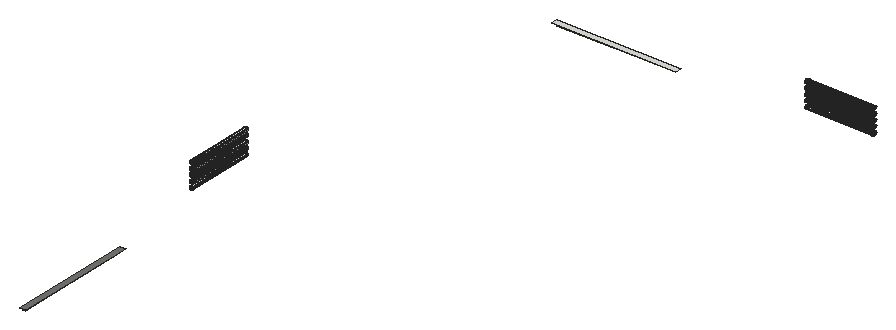
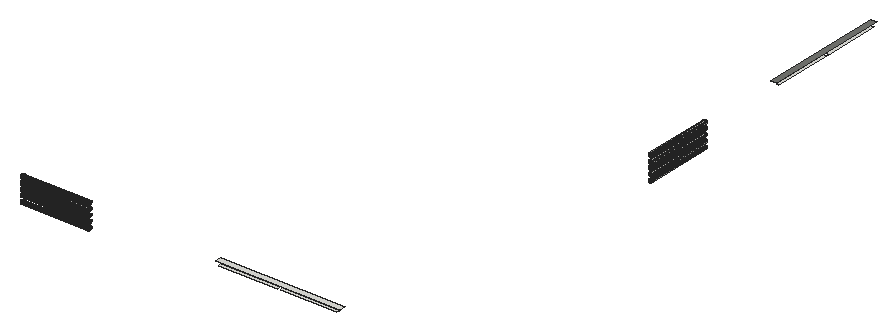
# SketchUp Ruby script. Lengths in inches.
U = 1.inch
M = Sketchup.active_model
def pt(a) = Geom::Point3d.new(a.map { |v| v * U })
def face(e, loops, mat)
  f = e.add_face(loops[0].map { |a| pt(a) })
  loops[1..].each { |l| e.add_face(l.map { |a| pt(a) }).erase! }
  f.material = f.back_material = mat if mat
  f
end
# faces: each face lists its corners as indices into pts; further lists are holes
def faces(e, pts, list, mat = nil) = list.each { |f| face(e, (f[0].is_a?(Array) ? f : [f]).map { |l| l.map { |i| pts[i] } }, mat) }
# xy, xz, yz: faces in a plane at the given z, y or x. An outline is a flat list of corners, or four numbers for a rectangle; further outlines are holes
def ring(l) = l.size == 4 ? [[l[0], l[1]], [l[2], l[1]], [l[2], l[3]], [l[0], l[3]]] : l.each_slice(2).to_a
def flat(e, list, mat, &to3) = list.each { |f| face(e, (f[0].is_a?(Array) ? f : [f]).map { |l| ring(l).map { |u, v| to3.(u, v) } }, mat) }
def xy(e, z, list, mat = nil) = flat(e, list, mat) { |x, y| [x, y, z] }
def xz(e, y, list, mat = nil) = flat(e, list, mat) { |x, z| [x, y, z] }
def yz(e, x, list, mat = nil) = flat(e, list, mat) { |y, z| [x, y, z] }
def lines(e, pts, list) = list.each { |a, b| e.add_line(pt(pts[a]), pt(pts[b])) }
# prism: a flat outline (further loops are holes) pulled along v
def prism(e, loops, v, mat = nil)
  f = face(e, loops, mat); d = Geom::Vector3d.new(v.map { |x| x * U })
  f.pushpull(f.normal.samedirection?(d) ? d.length : -d.length)
end
def box(e, o, s, mat = nil) = prism(e, [[o, [o[0] + s[0], o[1], o[2]], [o[0] + s[0], o[1] + s[1], o[2]], [o[0], o[1] + s[1], o[2]]]], [0, 0, s[2]], mat)
def at(x, y, z, deg = 0) = Geom::Transformation.translation(pt([x, y, z])) * Geom::Transformation.rotation(ORIGIN, Z_AXIS, deg.degrees)
def axes(o, x, y, z) = Geom::Transformation.new([*x, 0, *y, 0, *z, 0, *pt(o).to_a, 1])
def part(name) = M.definitions.add(name)
# library, detail: a bought-in or finely detailed component or shape, given as its bounding box
def library(name, o, s) = part(name).tap { |d| box(d.entities, o, s) }
def detail(e, o, s) = box(e.add_group.entities, o, s)
def put(e, d, t, mat = nil) = e.add_instance(d, t).tap { |i| i.material = mat if mat }
def group(e, t, mat = nil) = e.add_group.tap { |g| g.transformation = t; g.material = mat if mat }.entities
root = M.entities
M.materials.add("[Metal Seamed]").color = [118, 119, 115]
xy(root,1727.61,[[120,175.92,126,293.77],[120,299.77,126,423.61],[211.11,1458.8125,328.96,1464.8125],[334.96,1458.8125,458.8,1464.8125]])
xy(root,1733.61,[[205.11,1452.8125,464.8,1464.8125]])
xy(root,1733.61,[[120,169.92,132,429.61]],"[Metal Seamed]")
p = [[83.53,662.8,1725.02],[82.57,662.8,1725.14],[82.57,806.17,1725.14],[83.53,806.17,1725.02],[84.48,662.8,1725.14],[84.48,806.17,1725.14],
  [697.99,1500.33,1725.14],[697.99,1501.28,1725.02],[841.36,1501.28,1725.02],[841.36,1500.33,1725.14],[697.99,1502.24,1725.14],[841.36,1502.24,1725.14],
  [81.68,662.8,1725.51],[81.68,806.17,1725.51],[85.37,662.8,1725.51],[85.37,806.17,1725.51],[697.99,1499.44,1725.51],[841.36,1499.44,1725.51],
  [697.99,1503.13,1725.51],[841.36,1503.13,1725.51],[80.92,662.8,1726.1],[80.92,806.17,1726.1],[86.13,662.8,1726.1],[86.13,806.17,1726.1],
  [697.99,1498.68,1726.1],[841.36,1498.68,1726.1],[697.99,1503.89,1726.1],[841.36,1503.89,1726.1],[80.33,662.8,1726.86],[80.33,806.17,1726.86],
  [86.72,662.8,1726.86],[86.72,806.17,1726.86],[697.99,1498.09,1726.86],[841.36,1498.09,1726.86],[697.99,1504.48,1726.86],[841.36,1504.48,1726.86],
  [79.97,662.8,1727.75],[79.97,806.17,1727.75],[87.09,662.8,1727.75],[87.09,806.17,1727.75],[697.99,1497.72,1727.75],[841.36,1497.72,1727.75],
  [697.99,1504.85,1727.75],[841.36,1504.85,1727.75],[79.84,662.8,1728.7],[79.84,806.17,1728.7],[87.21,662.8,1728.7],[87.21,806.17,1728.7],
  [697.99,1497.6,1728.7],[841.36,1497.6,1728.7],[697.99,1504.97,1728.7],[841.36,1504.97,1728.7],[79.97,662.8,1729.66],[79.97,806.17,1729.66],
  [87.09,662.8,1729.66],[87.09,806.17,1729.66],[697.99,1497.72,1729.66],[841.36,1497.72,1729.66],[697.99,1504.85,1729.66],[841.36,1504.85,1729.66],
  [80.33,662.8,1730.55],[80.33,806.17,1730.55],[86.72,662.8,1730.55],[86.72,806.17,1730.55],[697.99,1498.09,1730.55],[841.36,1498.09,1730.55],
  [697.99,1504.48,1730.55],[841.36,1504.48,1730.55],[80.92,662.8,1731.3125],[80.92,806.17,1731.3125],[86.13,662.8,1731.3125],[86.13,806.17,1731.3125],
  [697.99,1498.68,1731.3125],[841.36,1498.68,1731.3125],[697.99,1503.89,1731.3125],[841.36,1503.89,1731.3125],[81.68,662.8,1731.9],[81.68,806.17,1731.9],
  [85.37,662.8,1731.9],[85.37,806.17,1731.9],[697.99,1499.44,1731.9],[841.36,1499.44,1731.9],[697.99,1503.13,1731.9],[841.36,1503.13,1731.9],
  [82.57,662.8,1732.27],[82.57,806.17,1732.27],[84.48,662.8,1732.27],[84.48,806.17,1732.27],[697.99,1500.33,1732.27],[841.36,1500.33,1732.27],
  [697.99,1502.24,1732.27],[841.36,1502.24,1732.27],[83.53,662.8,1732.39],[83.53,806.17,1732.39],[697.99,1501.28,1732.39],[841.36,1501.28,1732.39],
  [83.53,662.8,1737.02],[82.57,662.8,1737.14],[82.57,806.17,1737.14],[83.53,806.17,1737.02],[84.48,662.8,1737.14],[84.48,806.17,1737.14],
  [697.99,1500.33,1737.14],[697.99,1501.28,1737.02],[841.36,1501.28,1737.02],[841.36,1500.33,1737.14],[697.99,1502.24,1737.14],[841.36,1502.24,1737.14],
  [81.68,662.8,1737.51],[81.68,806.17,1737.51],[85.37,662.8,1737.51],[85.37,806.17,1737.51],[697.99,1499.44,1737.51],[841.36,1499.44,1737.51],
  [697.99,1503.13,1737.51],[841.36,1503.13,1737.51],[80.92,662.8,1738.1],[80.92,806.17,1738.1],[86.13,662.8,1738.1],[86.13,806.17,1738.1],
  [697.99,1498.68,1738.1],[841.36,1498.68,1738.1],[697.99,1503.89,1738.1],[841.36,1503.89,1738.1],[80.33,662.8,1738.86],[80.33,806.17,1738.86],
  [86.72,662.8,1738.86],[86.72,806.17,1738.86],[697.99,1498.09,1738.86],[841.36,1498.09,1738.86],[697.99,1504.48,1738.86],[841.36,1504.48,1738.86],
  [79.97,662.8,1739.75],[79.97,806.17,1739.75],[87.09,662.8,1739.75],[87.09,806.17,1739.75],[697.99,1497.72,1739.75],[841.36,1497.72,1739.75],
  [697.99,1504.85,1739.75],[841.36,1504.85,1739.75],[79.84,662.8,1740.7],[79.84,806.17,1740.7],[87.21,662.8,1740.7],[87.21,806.17,1740.7],
  [697.99,1497.6,1740.7],[841.36,1497.6,1740.7],[697.99,1504.97,1740.7],[841.36,1504.97,1740.7],[79.97,662.8,1741.66],[79.97,806.17,1741.66],
  [87.09,662.8,1741.66],[87.09,806.17,1741.66],[697.99,1497.72,1741.66],[841.36,1497.72,1741.66],[697.99,1504.85,1741.66],[841.36,1504.85,1741.66],
  [80.33,662.8,1742.55],[80.33,806.17,1742.55],[86.72,662.8,1742.55],[86.72,806.17,1742.55],[697.99,1498.09,1742.55],[841.36,1498.09,1742.55],
  [697.99,1504.48,1742.55],[841.36,1504.48,1742.55],[80.92,662.8,1743.3125],[80.92,806.17,1743.3125],[86.13,662.8,1743.3125],[86.13,806.17,1743.3125],
  [697.99,1498.68,1743.3125],[841.36,1498.68,1743.3125],[697.99,1503.89,1743.3125],[841.36,1503.89,1743.3125],[81.68,662.8,1743.9],[81.68,806.17,1743.9],
  [85.37,662.8,1743.9],[85.37,806.17,1743.9],[697.99,1499.44,1743.9],[841.36,1499.44,1743.9],[697.99,1503.13,1743.9],[841.36,1503.13,1743.9],
  [82.57,662.8,1744.27],[82.57,806.17,1744.27],[84.48,662.8,1744.27],[84.48,806.17,1744.27],[697.99,1500.33,1744.27],[841.36,1500.33,1744.27],
  [697.99,1502.24,1744.27],[841.36,1502.24,1744.27],[83.53,662.8,1744.39],[83.53,806.17,1744.39],[697.99,1501.28,1744.39],[841.36,1501.28,1744.39],
  [83.53,662.8,1749.02],[82.57,662.8,1749.14],[82.57,806.17,1749.14],[83.53,806.17,1749.02],[84.48,662.8,1749.14],[84.48,806.17,1749.14],
  [697.99,1500.33,1749.14],[697.99,1501.28,1749.02],[841.36,1501.28,1749.02],[841.36,1500.33,1749.14],[697.99,1502.24,1749.14],[841.36,1502.24,1749.14],
  [81.68,662.8,1749.51],[81.68,806.17,1749.51],[85.37,662.8,1749.51],[85.37,806.17,1749.51],[697.99,1499.44,1749.51],[841.36,1499.44,1749.51],
  [697.99,1503.13,1749.51],[841.36,1503.13,1749.51],[80.92,662.8,1750.1],[80.92,806.17,1750.1],[86.13,662.8,1750.1],[86.13,806.17,1750.1],
  [697.99,1498.68,1750.1],[841.36,1498.68,1750.1],[697.99,1503.89,1750.1],[841.36,1503.89,1750.1],[80.33,662.8,1750.86],[80.33,806.17,1750.86],
  [86.72,662.8,1750.86],[86.72,806.17,1750.86],[697.99,1498.09,1750.86],[841.36,1498.09,1750.86],[697.99,1504.48,1750.86],[841.36,1504.48,1750.86],
  [79.97,662.8,1751.75],[79.97,806.17,1751.75],[87.09,662.8,1751.75],[87.09,806.17,1751.75],[697.99,1497.72,1751.75],[841.36,1497.72,1751.75],
  [697.99,1504.85,1751.75],[841.36,1504.85,1751.75],[79.84,662.8,1752.7],[79.84,806.17,1752.7],[87.21,662.8,1752.7],[87.21,806.17,1752.7],
  [697.99,1497.6,1752.7],[841.36,1497.6,1752.7],[697.99,1504.97,1752.7],[841.36,1504.97,1752.7],[79.97,662.8,1753.66],[79.97,806.17,1753.66],
  [87.09,662.8,1753.66],[87.09,806.17,1753.66],[697.99,1497.72,1753.66],[841.36,1497.72,1753.66],[697.99,1504.85,1753.66],[841.36,1504.85,1753.66],
  [80.33,662.8,1754.55],[80.33,806.17,1754.55],[86.72,662.8,1754.55],[86.72,806.17,1754.55],[697.99,1498.09,1754.55],[841.36,1498.09,1754.55],
  [697.99,1504.48,1754.55],[841.36,1504.48,1754.55],[80.92,662.8,1755.3125],[80.92,806.17,1755.3125],[86.13,662.8,1755.3125],[86.13,806.17,1755.3125],
  [697.99,1498.68,1755.3125],[841.36,1498.68,1755.3125],[697.99,1503.89,1755.3125],[841.36,1503.89,1755.3125],[81.68,662.8,1755.9],[81.68,806.17,1755.9],
  [85.37,662.8,1755.9],[85.37,806.17,1755.9],[697.99,1499.44,1755.9],[841.36,1499.44,1755.9],[697.99,1503.13,1755.9],[841.36,1503.13,1755.9],
  [82.57,662.8,1756.27],[82.57,806.17,1756.27],[84.48,662.8,1756.27],[84.48,806.17,1756.27],[697.99,1500.33,1756.27],[841.36,1500.33,1756.27],
  [697.99,1502.24,1756.27],[841.36,1502.24,1756.27],[83.53,662.8,1756.39],[83.53,806.17,1756.39],[697.99,1501.28,1756.39],[841.36,1501.28,1756.39],
  [83.53,662.8,1761.02],[82.57,662.8,1761.14],[82.57,806.17,1761.14],[83.53,806.17,1761.02],[84.48,662.8,1761.14],[84.48,806.17,1761.14],
  [697.99,1500.33,1761.14],[697.99,1501.28,1761.02],[841.36,1501.28,1761.02],[841.36,1500.33,1761.14],[697.99,1502.24,1761.14],[841.36,1502.24,1761.14],
  [81.68,662.8,1761.51],[81.68,806.17,1761.51],[85.37,662.8,1761.51],[85.37,806.17,1761.51],[697.99,1499.44,1761.51],[841.36,1499.44,1761.51],
  [697.99,1503.13,1761.51],[841.36,1503.13,1761.51],[80.92,662.8,1762.1],[80.92,806.17,1762.1],[86.13,662.8,1762.1],[86.13,806.17,1762.1],
  [697.99,1498.68,1762.1],[841.36,1498.68,1762.1],[697.99,1503.89,1762.1],[841.36,1503.89,1762.1],[80.33,662.8,1762.86],[80.33,806.17,1762.86],
  [86.72,662.8,1762.86],[86.72,806.17,1762.86],[697.99,1498.09,1762.86],[841.36,1498.09,1762.86],[697.99,1504.48,1762.86],[841.36,1504.48,1762.86],
  [79.97,662.8,1763.75],[79.97,806.17,1763.75],[87.09,662.8,1763.75],[87.09,806.17,1763.75],[697.99,1497.72,1763.75],[841.36,1497.72,1763.75],
  [697.99,1504.85,1763.75],[841.36,1504.85,1763.75],[79.84,662.8,1764.7],[79.84,806.17,1764.7],[87.21,662.8,1764.7],[87.21,806.17,1764.7],
  [697.99,1497.6,1764.7],[841.36,1497.6,1764.7],[697.99,1504.97,1764.7],[841.36,1504.97,1764.7],[79.97,662.8,1765.66],[79.97,806.17,1765.66],
  [87.09,662.8,1765.66],[87.09,806.17,1765.66],[697.99,1497.72,1765.66],[841.36,1497.72,1765.66],[697.99,1504.85,1765.66],[841.36,1504.85,1765.66],
  [80.33,662.8,1766.55],[80.33,806.17,1766.55],[86.72,662.8,1766.55],[86.72,806.17,1766.55],[697.99,1498.09,1766.55],[841.36,1498.09,1766.55],
  [697.99,1504.48,1766.55],[841.36,1504.48,1766.55],[80.92,662.8,1767.3125],[80.92,806.17,1767.3125],[86.13,662.8,1767.3125],[86.13,806.17,1767.3125],
  [697.99,1498.68,1767.3125],[841.36,1498.68,1767.3125],[697.99,1503.89,1767.3125],[841.36,1503.89,1767.3125],[81.68,662.8,1767.9],[81.68,806.17,1767.9],
  [85.37,662.8,1767.9],[85.37,806.17,1767.9],[697.99,1499.44,1767.9],[841.36,1499.44,1767.9],[697.99,1503.13,1767.9],[841.36,1503.13,1767.9],
  [82.57,662.8,1768.27],[82.57,806.17,1768.27],[84.48,662.8,1768.27],[84.48,806.17,1768.27],[697.99,1500.33,1768.27],[841.36,1500.33,1768.27],
  [697.99,1502.24,1768.27],[841.36,1502.24,1768.27],[83.53,662.8,1768.39],[83.53,806.17,1768.39],[697.99,1501.28,1768.39],[841.36,1501.28,1768.39],
  [83.53,662.8,1773.02],[82.57,662.8,1773.14],[82.57,806.17,1773.14],[83.53,806.17,1773.02],[84.48,662.8,1773.14],[84.48,806.17,1773.14],
  [697.99,1500.33,1773.14],[697.99,1501.28,1773.02],[841.36,1501.28,1773.02],[841.36,1500.33,1773.14],[697.99,1502.24,1773.14],[841.36,1502.24,1773.14],
  [81.68,662.8,1773.51],[81.68,806.17,1773.51],[85.37,662.8,1773.51],[85.37,806.17,1773.51],[697.99,1499.44,1773.51],[841.36,1499.44,1773.51],
  [697.99,1503.13,1773.51],[841.36,1503.13,1773.51],[80.92,662.8,1774.1],[80.92,806.17,1774.1],[86.13,662.8,1774.1],[86.13,806.17,1774.1],
  [697.99,1498.68,1774.1],[841.36,1498.68,1774.1],[697.99,1503.89,1774.1],[841.36,1503.89,1774.1],[80.33,662.8,1774.86],[80.33,806.17,1774.86],
  [86.72,662.8,1774.86],[86.72,806.17,1774.86],[697.99,1498.09,1774.86],[841.36,1498.09,1774.86],[697.99,1504.48,1774.86],[841.36,1504.48,1774.86],
  [79.97,662.8,1775.75],[79.97,806.17,1775.75],[87.09,662.8,1775.75],[87.09,806.17,1775.75],[697.99,1497.72,1775.75],[841.36,1497.72,1775.75],
  [697.99,1504.85,1775.75],[841.36,1504.85,1775.75],[79.84,662.8,1776.7],[79.84,806.17,1776.7],[87.21,662.8,1776.7],[87.21,806.17,1776.7],
  [697.99,1497.6,1776.7],[841.36,1497.6,1776.7],[697.99,1504.97,1776.7],[841.36,1504.97,1776.7],[79.97,662.8,1777.66],[79.97,806.17,1777.66],
  [87.09,662.8,1777.66],[87.09,806.17,1777.66],[697.99,1497.72,1777.66],[841.36,1497.72,1777.66],[697.99,1504.85,1777.66],[841.36,1504.85,1777.66],
  [80.33,662.8,1778.55],[80.33,806.17,1778.55],[86.72,662.8,1778.55],[86.72,806.17,1778.55],[697.99,1498.09,1778.55],[841.36,1498.09,1778.55],
  [697.99,1504.48,1778.55],[841.36,1504.48,1778.55],[80.92,662.8,1779.3125],[80.92,806.17,1779.3125],[86.13,662.8,1779.3125],[86.13,806.17,1779.3125],
  [697.99,1498.68,1779.3125],[841.36,1498.68,1779.3125],[697.99,1503.89,1779.3125],[841.36,1503.89,1779.3125],[81.68,662.8,1779.9],[81.68,806.17,1779.9],
  [85.37,662.8,1779.9],[85.37,806.17,1779.9],[697.99,1499.44,1779.9],[841.36,1499.44,1779.9],[697.99,1503.13,1779.9],[841.36,1503.13,1779.9],
  [82.57,662.8,1780.27],[82.57,806.17,1780.27],[84.48,662.8,1780.27],[84.48,806.17,1780.27],[697.99,1500.33,1780.27],[841.36,1500.33,1780.27],
  [697.99,1502.24,1780.27],[841.36,1502.24,1780.27],[83.53,662.8,1780.39],[83.53,806.17,1780.39],[697.99,1501.28,1780.39],[841.36,1501.28,1780.39]]
faces(root,p,[[0,1,2,3],[4,0,3,5],[6,7,8,9],[7,10,11,8],[1,12,13,2],[14,4,5,15],[16,6,9,17],[10,18,19,11],
  [12,20,21,13],[22,14,15,23],[24,16,17,25],[18,26,27,19],[20,28,29,21],[30,22,23,31],[32,24,25,33],[26,34,35,27],
  [28,36,37,29],[38,30,31,39],[40,32,33,41],[34,42,43,35],[36,44,45,37],[46,38,39,47],[48,40,41,49],[42,50,51,43],
  [44,52,53,45],[54,46,47,55],[56,48,49,57],[50,58,59,51],[52,60,61,53],[62,54,55,63],[64,56,57,65],[58,66,67,59],
  [60,68,69,61],[70,62,63,71],[72,64,65,73],[66,74,75,67],[68,76,77,69],[78,70,71,79],[80,72,73,81],[74,82,83,75],
  [76,84,85,77],[86,78,79,87],[88,80,81,89],[82,90,91,83],[84,92,93,85],[92,86,87,93],[94,88,89,95],[90,94,95,91],
  [96,97,98,99],[100,96,99,101],[102,103,104,105],[103,106,107,104],[97,108,109,98],[110,100,101,111],[112,102,105,113],[106,114,115,107],
  [108,116,117,109],[118,110,111,119],[120,112,113,121],[114,122,123,115],[116,124,125,117],[126,118,119,127],[128,120,121,129],[122,130,131,123],
  [124,132,133,125],[134,126,127,135],[136,128,129,137],[130,138,139,131],[132,140,141,133],[142,134,135,143],[144,136,137,145],[138,146,147,139],
  [140,148,149,141],[150,142,143,151],[152,144,145,153],[146,154,155,147],[148,156,157,149],[158,150,151,159],[160,152,153,161],[154,162,163,155],
  [156,164,165,157],[166,158,159,167],[168,160,161,169],[162,170,171,163],[164,172,173,165],[174,166,167,175],[176,168,169,177],[170,178,179,171],
  [172,180,181,173],[182,174,175,183],[184,176,177,185],[178,186,187,179],[180,188,189,181],[188,182,183,189],[190,184,185,191],[186,190,191,187],
  [192,193,194,195],[196,192,195,197],[198,199,200,201],[199,202,203,200],[193,204,205,194],[206,196,197,207],[208,198,201,209],[202,210,211,203],
  [204,212,213,205],[214,206,207,215],[216,208,209,217],[210,218,219,211],[212,220,221,213],[222,214,215,223],[224,216,217,225],[218,226,227,219],
  [220,228,229,221],[230,222,223,231],[232,224,225,233],[226,234,235,227],[228,236,237,229],[238,230,231,239],[240,232,233,241],[234,242,243,235],
  [236,244,245,237],[246,238,239,247],[248,240,241,249],[242,250,251,243],[244,252,253,245],[254,246,247,255],[256,248,249,257],[250,258,259,251],
  [252,260,261,253],[262,254,255,263],[264,256,257,265],[258,266,267,259],[260,268,269,261],[270,262,263,271],[272,264,265,273],[266,274,275,267],
  [268,276,277,269],[278,270,271,279],[280,272,273,281],[274,282,283,275],[276,284,285,277],[284,278,279,285],[286,280,281,287],[282,286,287,283],
  [288,289,290,291],[292,288,291,293],[294,295,296,297],[295,298,299,296],[289,300,301,290],[302,292,293,303],[304,294,297,305],[298,306,307,299],
  [300,308,309,301],[310,302,303,311],[312,304,305,313],[306,314,315,307],[308,316,317,309],[318,310,311,319],[320,312,313,321],[314,322,323,315],
  [316,324,325,317],[326,318,319,327],[328,320,321,329],[322,330,331,323],[324,332,333,325],[334,326,327,335],[336,328,329,337],[330,338,339,331],
  [332,340,341,333],[342,334,335,343],[344,336,337,345],[338,346,347,339],[340,348,349,341],[350,342,343,351],[352,344,345,353],[346,354,355,347],
  [348,356,357,349],[358,350,351,359],[360,352,353,361],[354,362,363,355],[356,364,365,357],[366,358,359,367],[368,360,361,369],[362,370,371,363],
  [364,372,373,365],[374,366,367,375],[376,368,369,377],[370,378,379,371],[372,380,381,373],[380,374,375,381],[382,376,377,383],[378,382,383,379],
  [384,385,386,387],[388,384,387,389],[390,391,392,393],[391,394,395,392],[385,396,397,386],[398,388,389,399],[400,390,393,401],[394,402,403,395],
  [396,404,405,397],[406,398,399,407],[408,400,401,409],[402,410,411,403],[404,412,413,405],[414,406,407,415],[416,408,409,417],[410,418,419,411],
  [412,420,421,413],[422,414,415,423],[424,416,417,425],[418,426,427,419],[420,428,429,421],[430,422,423,431],[432,424,425,433],[426,434,435,427],
  [428,436,437,429],[438,430,431,439],[440,432,433,441],[434,442,443,435],[436,444,445,437],[446,438,439,447],[448,440,441,449],[442,450,451,443],
  [444,452,453,445],[454,446,447,455],[456,448,449,457],[450,458,459,451],[452,460,461,453],[462,454,455,463],[464,456,457,465],[458,466,467,459],
  [460,468,469,461],[470,462,463,471],[472,464,465,473],[466,474,475,467],[468,476,477,469],[476,470,471,477],[478,472,473,479],[474,478,479,475]])
